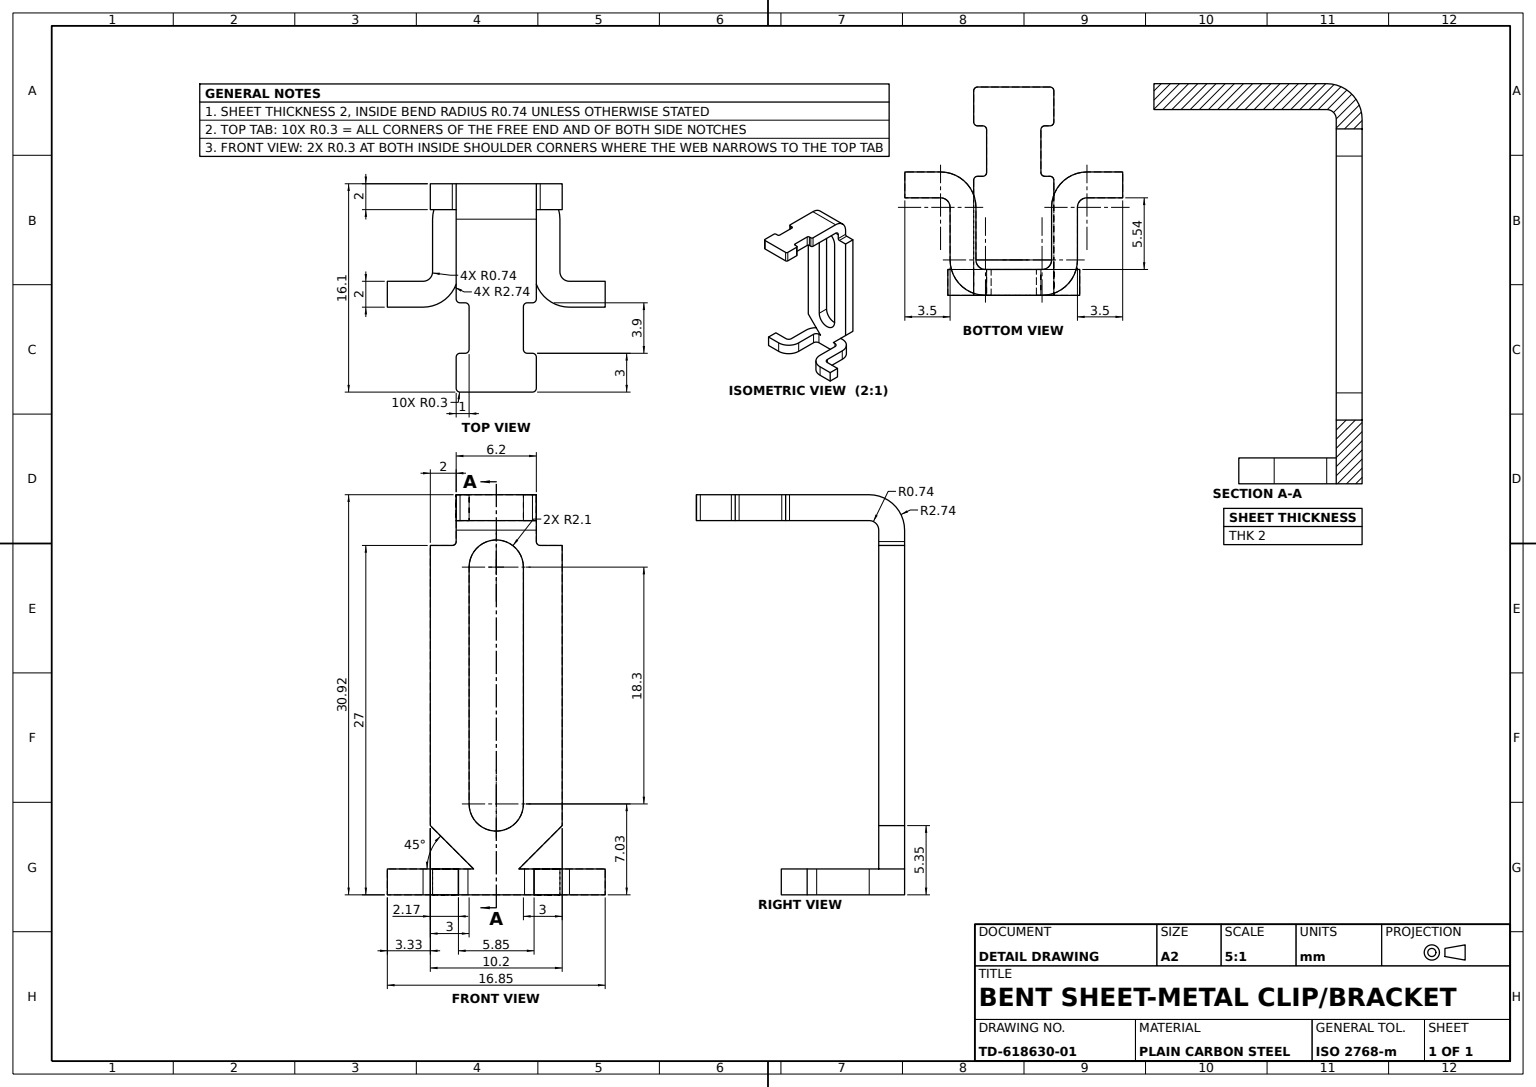
solid
v1 (5.1,10.825,-2)
v2 (5.1,10.825,0)
e1 v1 v2 LINE
v3 (5.1,-10.825,0)
e2 v3 v2 LINE
v4 (5.1,-10.825,-2)
e3 v4 v3 LINE
e4 v4 v1 LINE
face PLANE(AX(P(5.1,-10.825,-2),D(1,0,0),D(0,0,-1))) [e1 -e2 -e3 e4]
v5 (2.1,14.745,7.5)
v6 (2.4,14.745,7.2)
e5 v5 v6 CIRCLE(AX(P(2.4,14.745,7.5),D(0,-1,0),D(0,0,1)),0.3)
v7 (2.1,12.745,7.5)
e6 v7 v5 LINE
v8 (2.4,12.745,7.2)
e7 v8 v7 CIRCLE(AX(P(2.4,12.745,7.5),D(0,1,0),D(0,0,1)),0.3)
e8 v6 v8 LINE
face CYL(AX(P(2.4,14.745,7.5),D(0,1,0),D(0,0,1)),0.3) rev [-e5 -e6 -e7 -e8]
v9 (5.6616,-14.175,7.5366)
v10 (5.6616,-16.175,7.5366)
e9 v9 v10 LINE
v11 (2.925,-14.175,4.8)
e10 v11 v9 CIRCLE(AX(P(5.6616,-14.175,4.8),D(0,1,0),D(0,0,-1)),2.7366)
v12 (2.925,-16.175,4.8)
e11 v12 v11 LINE
e12 v10 v12 CIRCLE(AX(P(5.6616,-16.175,4.8),D(0,-1,0),D(0,0,-1)),2.7366)
face CYL(AX(P(5.6616,-16.175,4.8),D(0,-1,0),D(0,0,1)),2.7366) [-e9 -e10 -e11 -e12]
v13 (3.1,12.745,13.8)
v14 (2.8,12.745,14.1)
e13 v13 v14 CIRCLE(AX(P(2.8,12.745,13.8),D(0,-1,0),D(0,0,1)),0.3)
v15 (3.1,14.745,13.8)
e14 v15 v13 LINE
v16 (2.8,14.745,14.1)
e15 v16 v15 CIRCLE(AX(P(2.8,14.745,13.8),D(0,1,0),D(0,0,1)),0.3)
e16 v14 v16 LINE
face CYL(AX(P(2.8,14.745,13.8),D(0,-1,0),D(0,0,-1)),0.3) [-e13 -e14 -e15 -e16]
v17 (3.1,11.125,-2)
v18 (3.1,12.0084,-2)
e17 v17 v18 LINE
v19 (3.1,12.0084,0)
e18 v19 v18 LINE
v20 (3.1,11.125,0)
e19 v20 v19 LINE
e20 v20 v17 LINE
face PLANE(AX(P(3.1,10.825,-2),D(1,0,0),D(0,1,0))) [e17 -e18 -e19 e20]
v21 (-3.1,12.745,6.9)
v22 (-3.1,14.745,6.9)
e21 v21 v22 LINE
v23 (-2.8,12.745,7.2)
e22 v23 v21 CIRCLE(AX(P(-2.8,12.745,6.9),D(0,-1,0),D(0,0,1)),0.3)
v24 (-2.8,14.745,7.2)
e23 v24 v23 LINE
e24 v22 v24 CIRCLE(AX(P(-2.8,14.745,6.9),D(0,1,0),D(0,0,1)),0.3)
face CYL(AX(P(-2.8,14.745,6.9),D(0,1,0),D(0,0,1)),0.3) [-e21 -e22 -e23 -e24]
v25 (-1.75,-14.175,-2)
v26 (-1.75,-14.175,0)
e25 v25 v26 LINE
v27 (-2.1884,-14.175,-2)
e26 v25 v27 LINE
v28 (-2.1884,-14.175,0)
e27 v28 v27 LINE
e28 v26 v28 LINE
face PLANE(AX(P(-2.925,-14.175,-2),D(0,1,0),D(0,0,1))) [-e25 e26 -e27 -e28]
v29 (-4.925,-14.175,0.7366)
e29 v27 v29 CIRCLE(AX(P(-2.1884,-14.175,0.7366),D(0,1,0),D(0,0,-1)),2.7366)
v30 (-2.925,-14.175,0.7366)
e30 v30 v29 LINE
e31 v28 v30 CIRCLE(AX(P(-2.1884,-14.175,0.7366),D(0,1,0),D(0,0,-1)),0.7366)
face PLANE(AX(P(-2.1884,-14.175,0.7366),D(0,1,0),D(0,0,1))) [e27 e29 -e30 -e31]
v31 (-3.1,12.745,13.8)
v32 (-3.1,14.745,13.8)
e32 v31 v32 LINE
v33 (-2.8,12.745,14.1)
e33 v33 v31 CIRCLE(AX(P(-2.8,12.745,13.8),D(0,-1,0),D(0,0,1)),0.3)
v34 (-2.8,14.745,14.1)
e34 v34 v33 LINE
e35 v32 v34 CIRCLE(AX(P(-2.8,14.745,13.8),D(0,1,0),D(0,0,1)),0.3)
face CYL(AX(P(-2.8,14.745,13.8),D(0,-1,0),D(0,0,-1)),0.3) [-e32 -e33 -e34 -e35]
v35 (2.8,12.745,11.1)
v36 (3.1,12.745,11.4)
e36 v35 v36 CIRCLE(AX(P(2.8,12.745,11.4),D(0,-1,0),D(0,0,1)),0.3)
v37 (2.8,14.745,11.1)
e37 v37 v35 LINE
v38 (3.1,14.745,11.4)
e38 v38 v37 CIRCLE(AX(P(2.8,14.745,11.4),D(0,1,0),D(0,0,1)),0.3)
e39 v36 v38 LINE
face CYL(AX(P(2.8,14.745,11.4),D(0,1,0),D(0,0,1)),0.3) [-e36 -e37 -e38 -e39]
v39 (-3.1,14.745,0.7366)
e40 v22 v39 LINE
v40 (-3.1,12.745,0.7366)
e41 v40 v39 LINE
e42 v21 v40 LINE
face PLANE(AX(P(-3.1,14.745,0),D(-1,0,0),D(0,0,1))) [e21 e40 -e41 -e42]
v41 (-2.4,14.745,11.1)
v42 (-2.8,14.745,11.1)
e43 v41 v42 LINE
v43 (-3.1,14.745,11.4)
e44 v42 v43 CIRCLE(AX(P(-2.8,14.745,11.4),D(0,1,0),D(0,0,1)),0.3)
e45 v32 v43 LINE
e46 v16 v34 LINE
e47 v38 v15 LINE
v44 (2.4,14.745,11.1)
e48 v37 v44 LINE
v45 (2.1,14.745,10.8)
e49 v44 v45 CIRCLE(AX(P(2.4,14.745,10.8),D(0,-1,0),D(0,0,1)),0.3)
e50 v45 v5 LINE
v46 (2.8,14.745,7.2)
e51 v6 v46 LINE
v47 (3.1,14.745,6.9)
e52 v46 v47 CIRCLE(AX(P(2.8,14.745,6.9),D(0,1,0),D(0,0,1)),0.3)
v48 (3.1,14.745,0.7366)
e53 v48 v47 LINE
e54 v48 v39 LINE
v49 (-2.4,14.745,7.2)
e55 v24 v49 LINE
v50 (-2.1,14.745,7.5)
e56 v49 v50 CIRCLE(AX(P(-2.4,14.745,7.5),D(0,-1,0),D(0,0,1)),0.3)
v51 (-2.1,14.745,10.8)
e57 v50 v51 LINE
e58 v51 v41 CIRCLE(AX(P(-2.4,14.745,10.8),D(0,-1,0),D(0,0,1)),0.3)
face PLANE(AX(P(0,14.745,0),D(0,1,0),D(0,0,1))) [e43 e44 -e45 e35 -e46 e15 -e47 e38 e48 e49 e50 e5 e51 e52 -e53 e54 -e40 e24 e55 e56 e57 e58]
v52 (3.4,10.825,-2)
v53 (3.4,10.825,0)
e59 v52 v53 LINE
e60 v2 v53 LINE
e61 v1 v52 LINE
face PLANE(AX(P(-5.1,10.825,-2),D(0,1,0),D(0,0,1))) [e59 -e60 -e1 e61]
v54 (-2.1,12.745,7.5)
e62 v50 v54 LINE
v55 (-2.4,12.745,7.2)
e63 v55 v49 LINE
e64 v54 v55 CIRCLE(AX(P(-2.4,12.745,7.5),D(0,1,0),D(0,0,1)),0.3)
face CYL(AX(P(-2.4,14.745,7.5),D(0,1,0),D(0,0,1)),0.3) rev [-e62 -e56 -e63 -e64]
v56 (8.425,-16.175,7.5366)
v57 (8.425,-16.175,5.5366)
e65 v56 v57 LINE
e66 v10 v56 LINE
v58 (5.6616,-16.175,5.5366)
e67 v58 v10 LINE
e68 v58 v57 LINE
face PLANE(AX(P(8.425,-16.175,7.5366),D(0,1,0),D(0,0,1))) rev [-e65 -e66 -e67 e68]
v59 (8.425,-14.175,7.5366)
e69 v56 v59 LINE
v60 (8.425,-14.175,5.5366)
e70 v57 v60 LINE
e71 v59 v60 LINE
face PLANE(AX(P(8.425,-14.175,7.5366),D(-1,0,0),D(0,0,1))) rev [-e69 e65 e70 -e71]
v61 (4.925,-14.175,4.8)
v62 (5.6616,-14.175,5.5366)
e72 v61 v62 CIRCLE(AX(P(5.6616,-14.175,4.8),D(0,1,0),D(0,0,-1)),0.7366)
e73 v61 v11 LINE
e74 v62 v9 LINE
face PLANE(AX(P(5.6616,-14.175,4.8),D(0,1,0),D(0,0,1))) [-e72 e73 e10 -e74]
v63 (2.1,-9.15,-2)
v64 (2.1,-9.15,0)
e75 v63 v64 LINE
v65 (-2.1,-9.15,-2)
e76 v65 v63 CIRCLE(AX(P(0,-9.15,-2),D(0,0,1),D(1,0,0)),2.1)
v66 (-2.1,-9.15,0)
e77 v65 v66 LINE
e78 v66 v64 CIRCLE(AX(P(0,-9.15,0),D(0,0,1),D(1,0,0)),2.1)
face CYL(AX(P(0,-9.15,-2),D(0,0,1),D(1,0,0)),2.1) rev [-e75 -e76 e77 e78]
v67 (2.1,12.745,10.8)
e79 v45 v67 LINE
e80 v67 v7 LINE
face PLANE(AX(P(2.1,14.745,11.1),D(-1,0,0),D(0,0,1))) rev [-e50 e79 e80 e6]
v68 (-3.1,12.0084,0)
e81 v68 v19 LINE
v69 (3.1,12.745,0.7366)
e82 v19 v69 CIRCLE(AX(P(3.1,12.0084,0.7366),D(1,0,0),D(0,0,1)),0.7366)
e83 v69 v40 LINE
e84 v40 v68 CIRCLE(AX(P(-3.1,12.0084,0.7366),D(-1,0,0),D(0,0,1)),0.7366)
face CYL(AX(P(-3.1,12.0084,0.7366),D(-1,0,0),D(0,1,0)),0.7366) rev [e81 e82 e83 e84]
v70 (2.4,12.745,11.1)
e85 v70 v44 LINE
e86 v67 v70 CIRCLE(AX(P(2.4,12.745,10.8),D(0,1,0),D(0,0,1)),0.3)
face CYL(AX(P(2.4,14.745,10.8),D(0,1,0),D(0,0,1)),0.3) rev [-e49 -e85 -e86 -e79]
v71 (-5.6616,-16.175,7.5366)
v72 (-5.6616,-14.175,7.5366)
e87 v71 v72 LINE
v73 (-2.925,-16.175,4.8)
e88 v73 v71 CIRCLE(AX(P(-5.6616,-16.175,4.8),D(0,-1,0),D(0,0,1)),2.7366)
v74 (-2.925,-14.175,4.8)
e89 v73 v74 LINE
e90 v72 v74 CIRCLE(AX(P(-5.6616,-14.175,4.8),D(0,1,0),D(0,0,1)),2.7366)
face CYL(AX(P(-5.6616,-14.175,4.8),D(0,1,0),D(0,0,1)),2.7366) [-e87 -e88 e89 -e90]
v75 (2.1884,-14.175,0)
v76 (1.75,-14.175,0)
e91 v75 v76 LINE
v77 (2.1884,-14.175,-2)
e92 v75 v77 LINE
v78 (1.75,-14.175,-2)
e93 v77 v78 LINE
e94 v78 v76 LINE
face PLANE(AX(P(-2.925,-14.175,-2),D(0,1,0),D(0,0,1))) [-e91 e92 e93 e94]
v79 (-2.1,9.15,-2)
e95 v79 v65 LINE
v80 (-2.1,9.15,0)
e96 v79 v80 LINE
e97 v80 v66 LINE
face PLANE(AX(P(-2.1,9.15,-2),D(-1,0,0),D(0,-1,0))) rev [-e95 e96 e97 -e77]
e98 v62 v58 LINE
v81 (4.925,-16.175,4.8)
e99 v58 v81 CIRCLE(AX(P(5.6616,-16.175,4.8),D(0,-1,0),D(0,0,-1)),0.7366)
e100 v81 v61 LINE
face CYL(AX(P(5.6616,-16.175,4.8),D(0,-1,0),D(0,0,1)),0.7366) rev [e72 e98 e99 e100]
v82 (-2.8,12.745,11.1)
e101 v82 v42 LINE
v83 (-2.4,12.745,11.1)
e102 v41 v83 LINE
e103 v83 v82 LINE
face PLANE(AX(P(-3.1,14.745,11.1),D(0,0,1),D(0,-1,0))) rev [e101 -e43 e102 e103]
e104 v36 v13 LINE
face PLANE(AX(P(3.1,14.745,14.1),D(1,0,0),D(0,0,-1))) [-e104 e39 e47 e14]
v84 (2.1,9.15,0)
e105 v64 v84 LINE
v85 (2.1,9.15,-2)
e106 v85 v84 LINE
e107 v63 v85 LINE
face PLANE(AX(P(2.1,9.15,-2),D(1,0,0),D(0,1,0))) rev [e75 e105 -e106 -e107]
v86 (-3.4,10.825,0)
v87 (-5.1,10.825,0)
e108 v86 v87 LINE
v88 (-3.4,10.825,-2)
e109 v86 v88 LINE
v89 (-5.1,10.825,-2)
e110 v88 v89 LINE
e111 v89 v87 LINE
face PLANE(AX(P(-5.1,10.825,-2),D(0,1,0),D(0,0,1))) [-e108 e109 e110 e111]
v90 (-5.6616,-16.175,5.5366)
v91 (-8.425,-16.175,5.5366)
e112 v90 v91 LINE
e113 v90 v71 LINE
v92 (-8.425,-16.175,7.5366)
e114 v71 v92 LINE
e115 v92 v91 LINE
face PLANE(AX(P(-8.425,-16.175,7.5366),D(0,-1,0),D(0,0,-1))) [-e112 e113 e114 e115]
e116 v60 v62 LINE
face PLANE(AX(P(0,0,5.5366),D(0,0,1),D(-1,0,0))) rev [-e116 -e70 -e68 -e98]
e117 v18 v48 CIRCLE(AX(P(3.1,12.0084,0.7366),D(1,0,0),D(0,0,1)),2.7366)
e118 v69 v48 LINE
face PLANE(AX(P(3.1,12.0084,0.7366),D(1,0,0),D(0,0,-1))) [e18 e117 -e118 -e82]
v93 (-5.1,-10.825,-2)
v94 (-5.1,-10.825,0)
e119 v93 v94 LINE
e120 v93 v25 LINE
e121 v94 v26 LINE
face PLANE(AX(P(-5.1,-10.825,-2),D(-0.707106781,-0.707106781,0),D(0.707106781,-0.707106781,0))) [-e119 e120 e25 -e121]
v95 (-2.1884,-16.175,-2)
v96 (2.1884,-16.175,-2)
e122 v95 v96 LINE
v97 (2.1884,-16.175,0)
e123 v97 v96 LINE
v98 (-2.1884,-16.175,0)
e124 v98 v97 LINE
e125 v98 v95 LINE
face PLANE(AX(P(-2.925,-16.175,-2),D(0,-1,0),D(0,0,-1))) [e122 -e123 -e124 e125]
e126 v84 v80 CIRCLE(AX(P(0,9.15,0),D(0,0,1),D(1,0,0)),2.1)
e127 v98 v28 LINE
e128 v75 v97 LINE
e129 v76 v3 LINE
e130 v53 v20 CIRCLE(AX(P(3.4,11.125,0),D(0,0,-1),D(-1,0,0)),0.3)
v99 (-3.1,11.125,0)
e131 v68 v99 LINE
e132 v99 v86 CIRCLE(AX(P(-3.4,11.125,0),D(0,0,-1),D(-1,0,0)),0.3)
e133 v87 v94 LINE
face PLANE(AX(P(0,0,0),D(0,0,-1),D(-1,0,0))) rev [-e97 -e126 -e105 -e78] [e28 -e127 e124 -e128 e91 e129 e2 e60 e130 e19 -e81 e131 e132 e108 e133 e121]
v100 (-8.425,-14.175,7.5366)
e134 v100 v72 LINE
e135 v92 v100 LINE
face PLANE(AX(P(0,0,7.5366),D(0,0,1),D(1,0,0))) [e87 -e134 -e135 -e114]
e136 v85 v79 CIRCLE(AX(P(0,9.15,-2),D(0,0,1),D(1,0,0)),2.1)
face CYL(AX(P(0,9.15,-2),D(0,0,1),D(1,0,0)),2.1) rev [e126 -e96 -e136 e106]
v101 (-4.925,-16.175,0.7366)
v102 (-4.925,-16.175,4.8)
e137 v101 v102 LINE
v103 (-4.925,-14.175,4.8)
e138 v102 v103 LINE
e139 v103 v29 LINE
e140 v101 v29 LINE
face PLANE(AX(P(-4.925,0,0),D(1,0,0),D(0,0,-1))) rev [e137 e138 e139 -e140]
v104 (-2.925,-16.175,0.7366)
e141 v104 v98 CIRCLE(AX(P(-2.1884,-16.175,0.7366),D(0,-1,0),D(0,0,-1)),0.7366)
e142 v104 v101 LINE
e143 v101 v95 CIRCLE(AX(P(-2.1884,-16.175,0.7366),D(0,-1,0),D(0,0,-1)),2.7366)
face PLANE(AX(P(-2.1884,-16.175,0.7366),D(0,1,0),D(0,0,1))) rev [-e141 e142 e143 -e125]
e144 v89 v93 LINE
face PLANE(AX(P(-5.1,-10.825,-2),D(-1,0,0),D(0,0,1))) [-e133 -e111 e144 e119]
v105 (-3.1,11.125,-2)
e145 v88 v105 CIRCLE(AX(P(-3.4,11.125,-2),D(0,0,1),D(-1,0,0)),0.3)
e146 v105 v99 LINE
face CYL(AX(P(-3.4,11.125,-2),D(0,0,-1),D(-1,0,0)),0.3) rev [-e145 -e109 -e132 -e146]
e147 v81 v12 LINE
face PLANE(AX(P(5.6616,-16.175,4.8),D(0,1,0),D(0,0,1))) rev [-e99 e67 e12 -e147]
v106 (2.925,-16.175,0.7366)
e148 v97 v106 CIRCLE(AX(P(2.1884,-16.175,0.7366),D(0,-1,0),D(0,0,1)),0.7366)
v107 (4.925,-16.175,0.7366)
e149 v96 v107 CIRCLE(AX(P(2.1884,-16.175,0.7366),D(0,-1,0),D(0,0,1)),2.7366)
e150 v106 v107 LINE
face PLANE(AX(P(2.1884,-16.175,0.7366),D(0,-1,0),D(0,0,-1))) [-e148 e123 e149 -e150]
e151 v103 v74 LINE
e152 v74 v30 LINE
face PLANE(AX(P(-4.925,-14.175,0),D(0,-1,0),D(0,0,-1))) rev [-e139 e151 e152 e30]
e153 v106 v12 LINE
e154 v107 v81 LINE
face PLANE(AX(P(4.925,-16.175,4.8),D(0,-1,0),D(0,0,-1))) [e147 -e153 e150 e154]
e155 v23 v55 LINE
face PLANE(AX(P(-3.1,14.745,7.2),D(0,0,-1),D(0,1,0))) rev [e63 -e55 e23 e155]
v108 (2.925,-14.175,0.7366)
e156 v106 v108 LINE
e157 v108 v75 CIRCLE(AX(P(2.1884,-14.175,0.7366),D(0,1,0),D(0,0,1)),0.7366)
face CYL(AX(P(2.1884,-14.175,0.7366),D(0,1,0),D(1,0,0)),0.7366) rev [e148 e156 e157 e128]
e158 v11 v108 LINE
face PLANE(AX(P(2.925,0,0),D(-1,0,0),D(0,0,-1))) [-e156 e153 e11 e158]
e159 v59 v9 LINE
face PLANE(AX(P(4.925,-14.175,7.5366),D(0,-1,0),D(0,0,-1))) rev [e71 e116 e74 -e159]
e160 v30 v104 LINE
face CYL(AX(P(-2.1884,-16.175,0.7366),D(0,-1,0),D(-1,0,0)),0.7366) rev [e160 e141 e127 e31]
v109 (-8.425,-14.175,5.5366)
e161 v100 v109 LINE
e162 v91 v109 LINE
face PLANE(AX(P(-8.425,-14.175,7.5366),D(-1,0,0),D(0,0,1))) [-e115 e135 e161 -e162]
v110 (4.925,-14.175,0.7366)
e163 v110 v107 LINE
e164 v61 v110 LINE
face PLANE(AX(P(4.925,0,0),D(-1,0,0),D(0,0,-1))) rev [-e154 -e163 -e164 -e100]
v111 (-3.1,12.0084,-2)
e165 v68 v111 LINE
e166 v111 v105 LINE
face PLANE(AX(P(-3.1,10.825,-2),D(-1,0,0),D(0,0,1))) [e146 -e131 e165 e166]
v112 (-3.1,12.745,11.4)
e167 v112 v82 CIRCLE(AX(P(-2.8,12.745,11.4),D(0,-1,0),D(0,0,1)),0.3)
e168 v43 v112 LINE
face CYL(AX(P(-2.8,14.745,11.4),D(0,1,0),D(0,0,1)),0.3) [-e44 -e101 -e167 -e168]
face PLANE(AX(P(0,0,7.5366),D(0,0,1),D(-1,0,0))) [e9 e66 e69 e159]
v113 (2.8,12.745,7.2)
e169 v8 v113 LINE
e170 v113 v46 LINE
face PLANE(AX(P(3.1,14.745,7.2),D(0,0,-1),D(0,1,0))) rev [e169 e170 -e51 e8]
v114 (-2.1,12.745,10.8)
e171 v114 v51 LINE
e172 v83 v114 CIRCLE(AX(P(-2.4,12.745,10.8),D(0,1,0),D(0,0,1)),0.3)
face CYL(AX(P(-2.4,14.745,10.8),D(0,1,0),D(0,0,1)),0.3) rev [-e58 -e171 -e172 -e102]
e173 v108 v110 LINE
face PLANE(AX(P(4.925,-14.175,0),D(0,1,0),D(0,0,1))) [-e173 -e158 -e73 e164]
e174 v17 v52 CIRCLE(AX(P(3.4,11.125,-2),D(0,0,1),D(-1,0,0)),0.3)
face CYL(AX(P(3.4,11.125,-2),D(0,0,-1),D(-1,0,0)),0.3) rev [-e59 -e174 -e20 -e130]
e175 v104 v73 LINE
e176 v102 v73 LINE
face PLANE(AX(P(-4.925,-16.175,4.8),D(0,1,0),D(0,0,1))) rev [-e142 e175 -e176 -e137]
e177 v31 v112 LINE
face PLANE(AX(P(-3.1,14.745,0),D(-1,0,0),D(0,0,1))) [e45 e168 -e177 e32]
e178 v39 v111 CIRCLE(AX(P(-3.1,12.0084,0.7366),D(-1,0,0),D(0,0,1)),2.7366)
e179 v111 v18 LINE
face CYL(AX(P(-3.1,12.0084,0.7366),D(-1,0,0),D(0,1,0)),2.7366) [-e178 -e54 -e117 -e179]
v115 (-5.6616,-14.175,5.5366)
e180 v109 v115 LINE
e181 v115 v72 LINE
face PLANE(AX(P(-4.925,-14.175,7.5366),D(0,1,0),D(0,0,1))) [-e180 -e161 e134 -e181]
e182 v54 v114 LINE
face PLANE(AX(P(-2.1,14.745,11.1),D(1,0,0),D(0,0,-1))) rev [-e57 e62 e182 e171]
e183 v78 v4 LINE
face PLANE(AX(P(5.1,-10.825,-2),D(0.707106781,-0.707106781,0),D(0.707106781,0.707106781,0))) [-e129 -e94 e183 e3]
e184 v90 v115 LINE
face PLANE(AX(P(0,0,5.5366),D(0,0,1),D(1,0,0))) rev [-e184 e112 e162 e180]
e185 v115 v103 CIRCLE(AX(P(-5.6616,-14.175,4.8),D(0,1,0),D(0,0,1)),0.7366)
face PLANE(AX(P(-5.6616,-14.175,4.8),D(0,-1,0),D(0,0,-1))) rev [e181 e90 -e151 -e185]
face PLANE(AX(P(-2.925,0,0),D(1,0,0),D(0,0,-1))) [-e175 -e160 -e152 -e89]
e186 v110 v77 CIRCLE(AX(P(2.1884,-14.175,0.7366),D(0,1,0),D(0,0,1)),2.7366)
face PLANE(AX(P(2.1884,-14.175,0.7366),D(0,-1,0),D(0,0,-1))) rev [e173 e186 -e92 -e157]
e187 v77 v96 LINE
e188 v95 v27 LINE
face PLANE(AX(P(0,0,-2),D(0,0,-1),D(-1,0,0))) [-e110 e145 -e166 e179 -e17 e174 -e61 -e4 -e183 -e93 e187 -e122 e188 -e26 -e120 -e144] [e95 e76 e107 e136]
e189 v35 v70 LINE
face PLANE(AX(P(3.1,14.745,11.1),D(0,0,1),D(0,-1,0))) rev [e189 e85 -e48 e37]
v116 (3.1,12.745,6.9)
e190 v47 v116 LINE
e191 v69 v116 LINE
face PLANE(AX(P(3.1,14.745,14.1),D(1,0,0),D(0,0,-1))) [e190 -e191 e118 e53]
e192 v116 v113 CIRCLE(AX(P(2.8,12.745,6.9),D(0,-1,0),D(0,0,1)),0.3)
face CYL(AX(P(2.8,14.745,6.9),D(0,1,0),D(0,0,1)),0.3) [-e192 -e190 -e52 -e170]
face CYL(AX(P(-2.1884,-16.175,0.7366),D(0,-1,0),D(-1,0,0)),2.7366) [-e29 -e188 -e143 e140]
face PLANE(AX(P(-3.1,12.0084,0.7366),D(1,0,0),D(0,0,-1))) rev [e41 e178 -e165 -e84]
e193 v14 v33 LINE
face PLANE(AX(P(-3.1,14.745,14.1),D(0,0,1),D(0,-1,0))) [e34 -e193 e16 e46]
e194 v102 v90 CIRCLE(AX(P(-5.6616,-16.175,4.8),D(0,-1,0),D(0,0,1)),0.7366)
face CYL(AX(P(-5.6616,-14.175,4.8),D(0,1,0),D(0,0,1)),0.7366) rev [e194 e184 e185 -e138]
face PLANE(AX(P(-5.6616,-16.175,4.8),D(0,-1,0),D(0,0,-1))) [e88 -e113 -e194 e176]
face CYL(AX(P(2.1884,-14.175,0.7366),D(0,1,0),D(1,0,0)),2.7366) [e163 -e149 -e187 -e186]
face PLANE(AX(P(0,12.745,0),D(0,1,0),D(0,0,1))) rev [e64 -e155 e22 e42 -e83 e191 e192 -e169 e7 -e80 e86 -e189 e36 e104 e13 e193 e33 e177 e167 -e103 e172 -e182]
